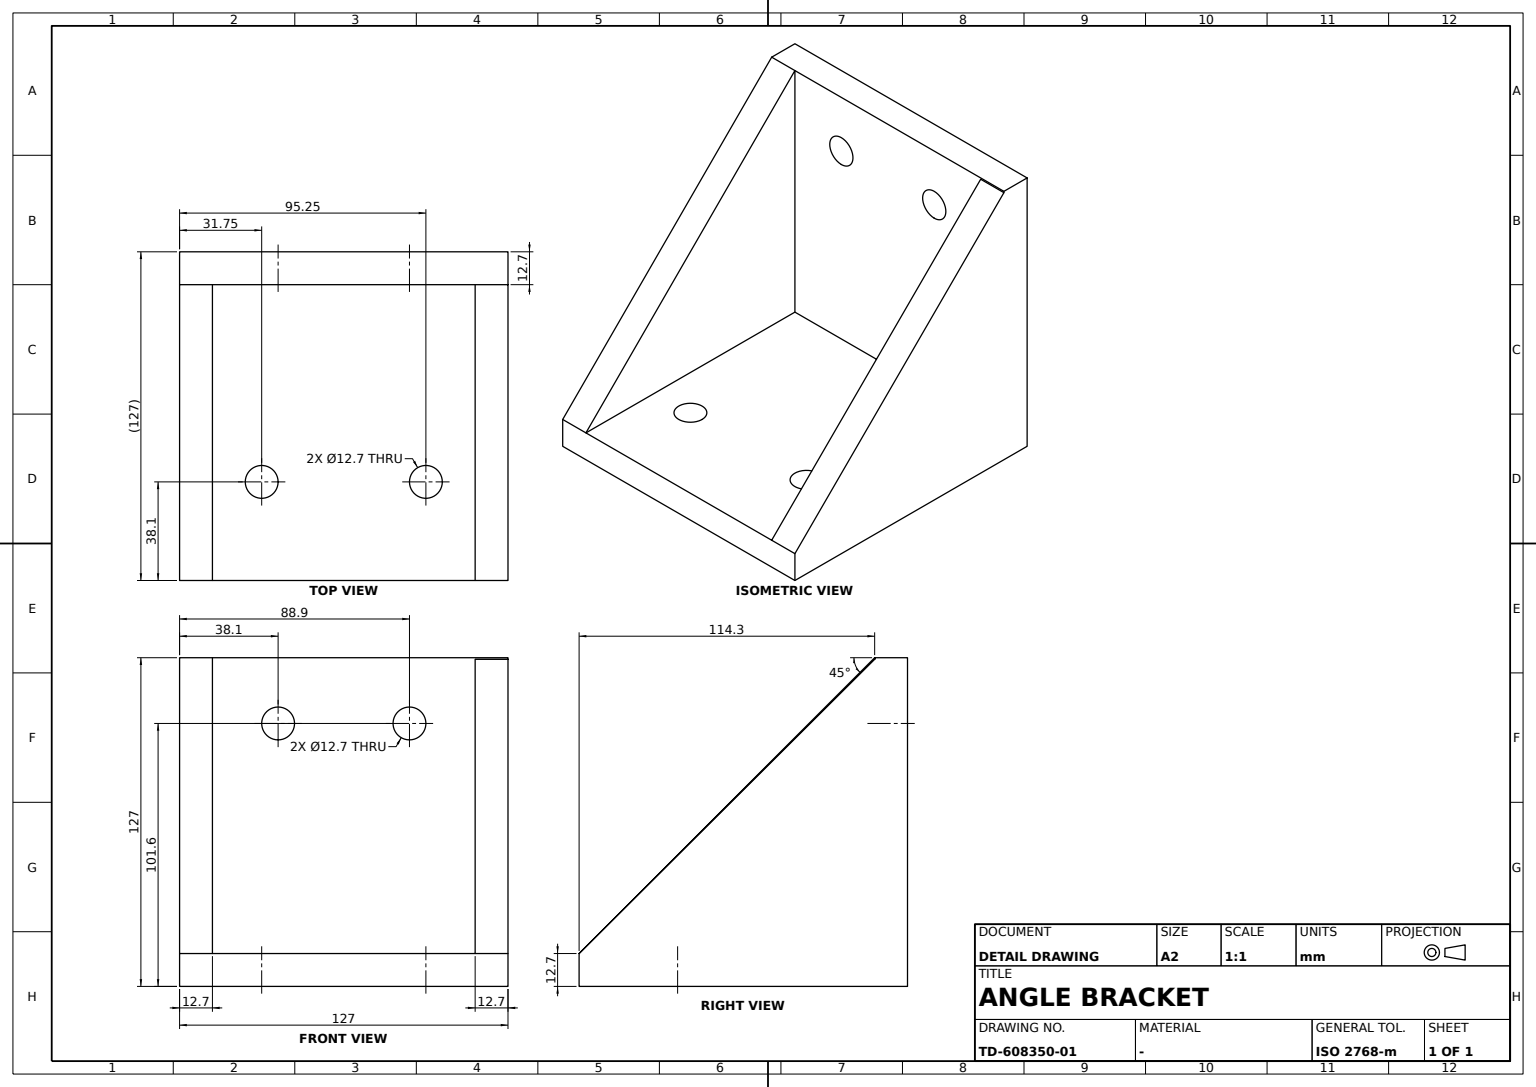
ISO-10303-21;
HEADER;
FILE_DESCRIPTION((''),'2;1');
FILE_NAME('','',(''),(''),'','','');
FILE_SCHEMA(('AUTOMOTIVE_DESIGN'));
ENDSEC;
DATA;
#1=APPLICATION_CONTEXT('');
#2=PRODUCT_CONTEXT('',#1,'mechanical');
#3=PRODUCT('','','',(#2));
#4=PRODUCT_DEFINITION_FORMATION('','',#3);
#5=PRODUCT_DEFINITION_CONTEXT('',#1,'design');
#6=PRODUCT_DEFINITION('','',#4,#5);
#7=PRODUCT_DEFINITION_SHAPE('','',#6);
#8=(LENGTH_UNIT()NAMED_UNIT(*)SI_UNIT(.MILLI.,.METRE.));
#9=(NAMED_UNIT(*)PLANE_ANGLE_UNIT()SI_UNIT($,.RADIAN.));
#10=(NAMED_UNIT(*)SI_UNIT($,.STERADIAN.)SOLID_ANGLE_UNIT());
#11=UNCERTAINTY_MEASURE_WITH_UNIT(LENGTH_MEASURE(0.005),#8,'distance_accuracy_value','');
#12=(GEOMETRIC_REPRESENTATION_CONTEXT(3)GLOBAL_UNCERTAINTY_ASSIGNED_CONTEXT((#11))GLOBAL_UNIT_ASSIGNED_CONTEXT((#8,#9,#10))REPRESENTATION_CONTEXT('',''));
#13=CARTESIAN_POINT('',(38.1,-25.4,0.));
#14=VERTEX_POINT('',#13);
#15=CARTESIAN_POINT('',(31.75,-25.4,0.));
#16=DIRECTION('',(0.,0.,1.));
#17=DIRECTION('',(1.,0.,0.));
#18=AXIS2_PLACEMENT_3D('',#15,#16,#17);
#19=CIRCLE('',#18,6.35);
#20=EDGE_CURVE('',#14,#14,#19,.T.);
#21=ORIENTED_EDGE('',*,*,#20,.F.);
#22=EDGE_LOOP('',(#21));
#23=FACE_BOUND('',#22,.T.);
#24=CARTESIAN_POINT('',(38.1,-25.4,12.7));
#25=VERTEX_POINT('',#24);
#26=CARTESIAN_POINT('',(31.75,-25.4,12.7));
#27=AXIS2_PLACEMENT_3D('',#26,#16,#17);
#28=CIRCLE('',#27,6.35);
#29=EDGE_CURVE('',#25,#25,#28,.T.);
#30=ORIENTED_EDGE('',*,*,#29,.T.);
#31=EDGE_LOOP('',(#30));
#32=FACE_BOUND('',#31,.T.);
#33=CARTESIAN_POINT('',(31.75,-25.4,6.35));
#34=AXIS2_PLACEMENT_3D('',#33,#16,#17);
#35=CYLINDRICAL_SURFACE('',#34,6.35);
#36=ADVANCED_FACE('',(#23,#32),#35,.F.);
#37=CARTESIAN_POINT('',(-25.4,50.8,107.95));
#38=VERTEX_POINT('',#37);
#39=CARTESIAN_POINT('',(-25.4,50.8,101.6));
#40=DIRECTION('',(0.,1.,0.));
#41=AXIS2_PLACEMENT_3D('',#39,#40,#16);
#42=CIRCLE('',#41,6.35);
#43=EDGE_CURVE('',#38,#38,#42,.F.);
#44=ORIENTED_EDGE('',*,*,#43,.T.);
#45=EDGE_LOOP('',(#44));
#46=FACE_BOUND('',#45,.T.);
#47=CARTESIAN_POINT('',(-25.4,63.5,95.25));
#48=VERTEX_POINT('',#47);
#49=CARTESIAN_POINT('',(-25.4,63.5,101.6));
#50=DIRECTION('',(0.,-1.,0.));
#51=DIRECTION('',(0.,0.,-1.));
#52=AXIS2_PLACEMENT_3D('',#49,#50,#51);
#53=CIRCLE('',#52,6.35);
#54=EDGE_CURVE('',#48,#48,#53,.T.);
#55=ORIENTED_EDGE('',*,*,#54,.F.);
#56=EDGE_LOOP('',(#55));
#57=FACE_BOUND('',#56,.T.);
#58=CARTESIAN_POINT('',(-25.4,57.81,101.6));
#59=AXIS2_PLACEMENT_3D('',#58,#50,#17);
#60=CYLINDRICAL_SURFACE('',#59,6.35);
#61=ADVANCED_FACE('',(#46,#57),#60,.F.);
#62=CARTESIAN_POINT('',(-63.5,50.8,127.));
#63=VERTEX_POINT('',#62);
#64=CARTESIAN_POINT('',(-50.8,50.8,127.));
#65=VERTEX_POINT('',#64);
#66=CARTESIAN_POINT('',(0.,50.8,127.));
#67=VECTOR('',#17,1000.);
#68=LINE('',#66,#67);
#69=EDGE_CURVE('',#63,#65,#68,.T.);
#70=ORIENTED_EDGE('',*,*,#69,.F.);
#71=CARTESIAN_POINT('',(-63.5,-63.5,12.7));
#72=VERTEX_POINT('',#71);
#73=CARTESIAN_POINT('',(-63.5,-69.85,6.35));
#74=DIRECTION('',(0.,-0.707106781,-0.707106781));
#75=VECTOR('',#74,1000.);
#76=LINE('',#73,#75);
#77=EDGE_CURVE('',#63,#72,#76,.T.);
#78=ORIENTED_EDGE('',*,*,#77,.T.);
#79=CARTESIAN_POINT('',(-50.8,-63.5,12.7));
#80=VERTEX_POINT('',#79);
#81=CARTESIAN_POINT('',(63.5,-63.5,12.7));
#82=LINE('',#81,#67);
#83=EDGE_CURVE('',#72,#80,#82,.T.);
#84=ORIENTED_EDGE('',*,*,#83,.T.);
#85=LINE('',#64,#75);
#86=EDGE_CURVE('',#65,#80,#85,.T.);
#87=ORIENTED_EDGE('',*,*,#86,.F.);
#88=EDGE_LOOP('',(#70,#78,#84,#87));
#89=FACE_BOUND('',#88,.T.);
#90=DIRECTION('',(0.,-0.707106781,0.707106781));
#91=AXIS2_PLACEMENT_3D('',#62,#90,#74);
#92=PLANE('',#91);
#93=ADVANCED_FACE('',(#89),#92,.T.);
#94=CARTESIAN_POINT('',(-25.4,-25.4,0.));
#95=VERTEX_POINT('',#94);
#96=CARTESIAN_POINT('',(-31.75,-25.4,0.));
#97=AXIS2_PLACEMENT_3D('',#96,#16,#17);
#98=CIRCLE('',#97,6.35);
#99=EDGE_CURVE('',#95,#95,#98,.T.);
#100=ORIENTED_EDGE('',*,*,#99,.T.);
#101=EDGE_LOOP('',(#100));
#102=FACE_BOUND('',#101,.T.);
#103=ORIENTED_EDGE('',*,*,#20,.T.);
#104=EDGE_LOOP('',(#103));
#105=FACE_BOUND('',#104,.T.);
#106=CARTESIAN_POINT('',(-63.5,-63.5,0.));
#107=VERTEX_POINT('',#106);
#108=CARTESIAN_POINT('',(-63.5,63.5,0.));
#109=VERTEX_POINT('',#108);
#110=CARTESIAN_POINT('',(-63.5,0.,0.));
#111=VECTOR('',#40,1000.);
#112=LINE('',#110,#111);
#113=EDGE_CURVE('',#107,#109,#112,.T.);
#114=ORIENTED_EDGE('',*,*,#113,.T.);
#115=CARTESIAN_POINT('',(63.5,63.5,0.));
#116=VERTEX_POINT('',#115);
#117=CARTESIAN_POINT('',(0.,63.5,0.));
#118=LINE('',#117,#67);
#119=EDGE_CURVE('',#109,#116,#118,.T.);
#120=ORIENTED_EDGE('',*,*,#119,.T.);
#121=CARTESIAN_POINT('',(63.5,-63.5,0.));
#122=VERTEX_POINT('',#121);
#123=CARTESIAN_POINT('',(63.5,0.,0.));
#124=VECTOR('',#50,1000.);
#125=LINE('',#123,#124);
#126=EDGE_CURVE('',#116,#122,#125,.T.);
#127=ORIENTED_EDGE('',*,*,#126,.T.);
#128=CARTESIAN_POINT('',(0.,-63.5,0.));
#129=DIRECTION('',(-1.,0.,0.));
#130=VECTOR('',#129,1000.);
#131=LINE('',#128,#130);
#132=EDGE_CURVE('',#122,#107,#131,.T.);
#133=ORIENTED_EDGE('',*,*,#132,.T.);
#134=EDGE_LOOP('',(#114,#120,#127,#133));
#135=FACE_BOUND('',#134,.T.);
#136=CARTESIAN_POINT('',(0.,0.,0.));
#137=AXIS2_PLACEMENT_3D('',#136,#16,#17);
#138=PLANE('',#137);
#139=ADVANCED_FACE('',(#102,#105,#135),#138,.F.);
#140=ORIENTED_EDGE('',*,*,#54,.T.);
#141=EDGE_LOOP('',(#140));
#142=FACE_BOUND('',#141,.T.);
#143=CARTESIAN_POINT('',(25.4,63.5,95.25));
#144=VERTEX_POINT('',#143);
#145=CARTESIAN_POINT('',(25.4,63.5,101.6));
#146=AXIS2_PLACEMENT_3D('',#145,#50,#51);
#147=CIRCLE('',#146,6.35);
#148=EDGE_CURVE('',#144,#144,#147,.T.);
#149=ORIENTED_EDGE('',*,*,#148,.T.);
#150=EDGE_LOOP('',(#149));
#151=FACE_BOUND('',#150,.T.);
#152=CARTESIAN_POINT('',(63.5,63.5,127.));
#153=VERTEX_POINT('',#152);
#154=VECTOR('',#16,1000.);
#155=LINE('',#115,#154);
#156=EDGE_CURVE('',#116,#153,#155,.T.);
#157=ORIENTED_EDGE('',*,*,#156,.F.);
#158=ORIENTED_EDGE('',*,*,#119,.F.);
#159=CARTESIAN_POINT('',(-63.5,63.5,127.));
#160=VERTEX_POINT('',#159);
#161=LINE('',#108,#154);
#162=EDGE_CURVE('',#109,#160,#161,.T.);
#163=ORIENTED_EDGE('',*,*,#162,.T.);
#164=CARTESIAN_POINT('',(0.,63.5,127.));
#165=LINE('',#164,#67);
#166=EDGE_CURVE('',#160,#153,#165,.T.);
#167=ORIENTED_EDGE('',*,*,#166,.T.);
#168=EDGE_LOOP('',(#157,#158,#163,#167));
#169=FACE_BOUND('',#168,.T.);
#170=AXIS2_PLACEMENT_3D('',#108,#50,#17);
#171=PLANE('',#170);
#172=ADVANCED_FACE('',(#142,#151,#169),#171,.F.);
#173=ORIENTED_EDGE('',*,*,#99,.F.);
#174=EDGE_LOOP('',(#173));
#175=FACE_BOUND('',#174,.T.);
#176=CARTESIAN_POINT('',(-25.4,-25.4,12.7));
#177=VERTEX_POINT('',#176);
#178=CARTESIAN_POINT('',(-31.75,-25.4,12.7));
#179=AXIS2_PLACEMENT_3D('',#178,#16,#17);
#180=CIRCLE('',#179,6.35);
#181=EDGE_CURVE('',#177,#177,#180,.T.);
#182=ORIENTED_EDGE('',*,*,#181,.T.);
#183=EDGE_LOOP('',(#182));
#184=FACE_BOUND('',#183,.T.);
#185=CARTESIAN_POINT('',(-31.75,-25.4,6.35));
#186=AXIS2_PLACEMENT_3D('',#185,#16,#17);
#187=CYLINDRICAL_SURFACE('',#186,6.35);
#188=ADVANCED_FACE('',(#175,#184),#187,.F.);
#189=LINE('',#106,#154);
#190=EDGE_CURVE('',#107,#72,#189,.T.);
#191=ORIENTED_EDGE('',*,*,#190,.T.);
#192=ORIENTED_EDGE('',*,*,#77,.F.);
#193=CARTESIAN_POINT('',(-63.5,0.,127.));
#194=LINE('',#193,#111);
#195=EDGE_CURVE('',#63,#160,#194,.T.);
#196=ORIENTED_EDGE('',*,*,#195,.T.);
#197=ORIENTED_EDGE('',*,*,#162,.F.);
#198=ORIENTED_EDGE('',*,*,#113,.F.);
#199=EDGE_LOOP('',(#191,#192,#196,#197,#198));
#200=FACE_BOUND('',#199,.T.);
#201=AXIS2_PLACEMENT_3D('',#106,#17,#40);
#202=PLANE('',#201);
#203=ADVANCED_FACE('',(#200),#202,.F.);
#204=CARTESIAN_POINT('',(50.8,-63.5,12.7));
#205=VERTEX_POINT('',#204);
#206=CARTESIAN_POINT('',(50.8,50.8,126.380035));
#207=VERTEX_POINT('',#206);
#208=DIRECTION('',(0.,0.709027052,0.705181281));
#209=VECTOR('',#208,1000.);
#210=LINE('',#204,#209);
#211=EDGE_CURVE('',#205,#207,#210,.T.);
#212=ORIENTED_EDGE('',*,*,#211,.T.);
#213=CARTESIAN_POINT('',(50.8,50.8,12.7));
#214=VERTEX_POINT('',#213);
#215=VECTOR('',#51,1000.);
#216=LINE('',#213,#215);
#217=EDGE_CURVE('',#207,#214,#216,.T.);
#218=ORIENTED_EDGE('',*,*,#217,.T.);
#219=CARTESIAN_POINT('',(50.8,0.,12.7));
#220=LINE('',#219,#124);
#221=EDGE_CURVE('',#214,#205,#220,.T.);
#222=ORIENTED_EDGE('',*,*,#221,.T.);
#223=EDGE_LOOP('',(#212,#218,#222));
#224=FACE_BOUND('',#223,.T.);
#225=CARTESIAN_POINT('',(50.8,0.,0.));
#226=AXIS2_PLACEMENT_3D('',#225,#17,#40);
#227=PLANE('',#226);
#228=ADVANCED_FACE('',(#224),#227,.F.);
#229=ORIENTED_EDGE('',*,*,#221,.F.);
#230=CARTESIAN_POINT('',(-50.8,50.8,12.7));
#231=VERTEX_POINT('',#230);
#232=CARTESIAN_POINT('',(0.,50.8,12.7));
#233=LINE('',#232,#130);
#234=EDGE_CURVE('',#214,#231,#233,.T.);
#235=ORIENTED_EDGE('',*,*,#234,.T.);
#236=CARTESIAN_POINT('',(-50.8,0.,12.7));
#237=LINE('',#236,#111);
#238=EDGE_CURVE('',#80,#231,#237,.T.);
#239=ORIENTED_EDGE('',*,*,#238,.F.);
#240=CARTESIAN_POINT('',(0.,-63.5,12.7));
#241=LINE('',#240,#130);
#242=EDGE_CURVE('',#205,#80,#241,.T.);
#243=ORIENTED_EDGE('',*,*,#242,.F.);
#244=EDGE_LOOP('',(#229,#235,#239,#243));
#245=FACE_BOUND('',#244,.T.);
#246=ORIENTED_EDGE('',*,*,#181,.F.);
#247=EDGE_LOOP('',(#246));
#248=FACE_BOUND('',#247,.T.);
#249=ORIENTED_EDGE('',*,*,#29,.F.);
#250=EDGE_LOOP('',(#249));
#251=FACE_BOUND('',#250,.T.);
#252=CARTESIAN_POINT('',(0.,0.,12.7));
#253=AXIS2_PLACEMENT_3D('',#252,#16,#17);
#254=PLANE('',#253);
#255=ADVANCED_FACE('',(#245,#248,#251),#254,.T.);
#256=ORIENTED_EDGE('',*,*,#148,.F.);
#257=EDGE_LOOP('',(#256));
#258=FACE_BOUND('',#257,.T.);
#259=CARTESIAN_POINT('',(25.4,50.8,107.95));
#260=VERTEX_POINT('',#259);
#261=CARTESIAN_POINT('',(25.4,50.8,101.6));
#262=AXIS2_PLACEMENT_3D('',#261,#40,#16);
#263=CIRCLE('',#262,6.35);
#264=EDGE_CURVE('',#260,#260,#263,.F.);
#265=ORIENTED_EDGE('',*,*,#264,.T.);
#266=EDGE_LOOP('',(#265));
#267=FACE_BOUND('',#266,.T.);
#268=CARTESIAN_POINT('',(25.4,57.81,101.6));
#269=AXIS2_PLACEMENT_3D('',#268,#50,#17);
#270=CYLINDRICAL_SURFACE('',#269,6.35);
#271=ADVANCED_FACE('',(#258,#267),#270,.F.);
#272=ORIENTED_EDGE('',*,*,#211,.F.);
#273=VERTEX_POINT('',#81);
#274=LINE('',#81,#130);
#275=EDGE_CURVE('',#273,#205,#274,.T.);
#276=ORIENTED_EDGE('',*,*,#275,.F.);
#277=CARTESIAN_POINT('',(63.5,50.8,126.380035));
#278=VERTEX_POINT('',#277);
#279=CARTESIAN_POINT('',(63.5,-6.004547,69.883597));
#280=LINE('',#279,#209);
#281=EDGE_CURVE('',#273,#278,#280,.T.);
#282=ORIENTED_EDGE('',*,*,#281,.T.);
#283=LINE('',#277,#130);
#284=EDGE_CURVE('',#278,#207,#283,.T.);
#285=ORIENTED_EDGE('',*,*,#284,.T.);
#286=EDGE_LOOP('',(#272,#276,#282,#285));
#287=FACE_BOUND('',#286,.T.);
#288=DIRECTION('',(0.,-0.705181281,0.709027052));
#289=AXIS2_PLACEMENT_3D('',#81,#288,#208);
#290=PLANE('',#289);
#291=ADVANCED_FACE('',(#287),#290,.T.);
#292=ORIENTED_EDGE('',*,*,#126,.F.);
#293=ORIENTED_EDGE('',*,*,#156,.T.);
#294=CARTESIAN_POINT('',(63.5,50.8,127.));
#295=VERTEX_POINT('',#294);
#296=CARTESIAN_POINT('',(63.5,0.,127.));
#297=LINE('',#296,#124);
#298=EDGE_CURVE('',#153,#295,#297,.T.);
#299=ORIENTED_EDGE('',*,*,#298,.T.);
#300=CARTESIAN_POINT('',(63.5,50.8,12.7));
#301=LINE('',#300,#154);
#302=EDGE_CURVE('',#278,#295,#301,.T.);
#303=ORIENTED_EDGE('',*,*,#302,.F.);
#304=ORIENTED_EDGE('',*,*,#281,.F.);
#305=LINE('',#121,#154);
#306=EDGE_CURVE('',#122,#273,#305,.T.);
#307=ORIENTED_EDGE('',*,*,#306,.F.);
#308=EDGE_LOOP('',(#292,#293,#299,#303,#304,#307));
#309=FACE_BOUND('',#308,.T.);
#310=AXIS2_PLACEMENT_3D('',#115,#129,#50);
#311=PLANE('',#310);
#312=ADVANCED_FACE('',(#309),#311,.F.);
#313=ORIENTED_EDGE('',*,*,#306,.T.);
#314=ORIENTED_EDGE('',*,*,#275,.T.);
#315=ORIENTED_EDGE('',*,*,#242,.T.);
#316=ORIENTED_EDGE('',*,*,#83,.F.);
#317=ORIENTED_EDGE('',*,*,#190,.F.);
#318=ORIENTED_EDGE('',*,*,#132,.F.);
#319=EDGE_LOOP('',(#313,#314,#315,#316,#317,#318));
#320=FACE_BOUND('',#319,.T.);
#321=AXIS2_PLACEMENT_3D('',#121,#40,#129);
#322=PLANE('',#321);
#323=ADVANCED_FACE('',(#320),#322,.F.);
#324=ORIENTED_EDGE('',*,*,#86,.T.);
#325=ORIENTED_EDGE('',*,*,#238,.T.);
#326=LINE('',#230,#154);
#327=EDGE_CURVE('',#231,#65,#326,.T.);
#328=ORIENTED_EDGE('',*,*,#327,.T.);
#329=EDGE_LOOP('',(#324,#325,#328));
#330=FACE_BOUND('',#329,.T.);
#331=CARTESIAN_POINT('',(-50.8,0.,0.));
#332=AXIS2_PLACEMENT_3D('',#331,#129,#50);
#333=PLANE('',#332);
#334=ADVANCED_FACE('',(#330),#333,.F.);
#335=ORIENTED_EDGE('',*,*,#264,.F.);
#336=EDGE_LOOP('',(#335));
#337=FACE_BOUND('',#336,.T.);
#338=ORIENTED_EDGE('',*,*,#302,.T.);
#339=LINE('',#66,#130);
#340=EDGE_CURVE('',#295,#65,#339,.T.);
#341=ORIENTED_EDGE('',*,*,#340,.T.);
#342=ORIENTED_EDGE('',*,*,#327,.F.);
#343=ORIENTED_EDGE('',*,*,#234,.F.);
#344=ORIENTED_EDGE('',*,*,#217,.F.);
#345=ORIENTED_EDGE('',*,*,#284,.F.);
#346=EDGE_LOOP('',(#338,#341,#342,#343,#344,#345));
#347=FACE_BOUND('',#346,.T.);
#348=ORIENTED_EDGE('',*,*,#43,.F.);
#349=EDGE_LOOP('',(#348));
#350=FACE_BOUND('',#349,.T.);
#351=AXIS2_PLACEMENT_3D('',#300,#40,#129);
#352=PLANE('',#351);
#353=ADVANCED_FACE('',(#337,#347,#350),#352,.F.);
#354=ORIENTED_EDGE('',*,*,#298,.F.);
#355=ORIENTED_EDGE('',*,*,#166,.F.);
#356=ORIENTED_EDGE('',*,*,#195,.F.);
#357=ORIENTED_EDGE('',*,*,#69,.T.);
#358=ORIENTED_EDGE('',*,*,#340,.F.);
#359=EDGE_LOOP('',(#354,#355,#356,#357,#358));
#360=FACE_BOUND('',#359,.T.);
#361=CARTESIAN_POINT('',(0.,0.,127.));
#362=AXIS2_PLACEMENT_3D('',#361,#16,#17);
#363=PLANE('',#362);
#364=ADVANCED_FACE('',(#360),#363,.T.);
#365=CLOSED_SHELL('',(#36,#61,#93,#139,#172,#188,#203,#228,#255,#271,#291,#312,#323,#334,#353,#364));
#366=MANIFOLD_SOLID_BREP('',#365);
#367=ADVANCED_BREP_SHAPE_REPRESENTATION('',(#366),#12);
#368=SHAPE_DEFINITION_REPRESENTATION(#7,#367);
ENDSEC;
END-ISO-10303-21;
